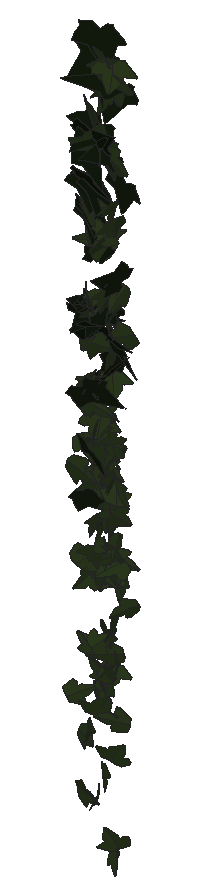
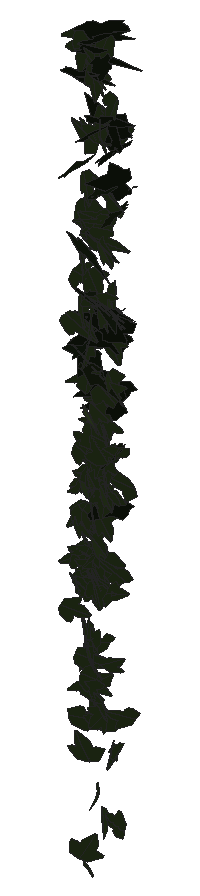
# SketchUp Ruby script. Lengths in inches.
U = 1.inch
M = Sketchup.active_model
def pt(a) = Geom::Point3d.new(a.map { |v| v * U })
def face(e, loops, mat)
  f = e.add_face(loops[0].map { |a| pt(a) })
  loops[1..].each { |l| e.add_face(l.map { |a| pt(a) }).erase! }
  f.material = f.back_material = mat if mat
  f
end
# faces: each face lists its corners as indices into pts; further lists are holes
def faces(e, pts, list, mat = nil) = list.each { |f| face(e, (f[0].is_a?(Array) ? f : [f]).map { |l| l.map { |i| pts[i] } }, mat) }
# xy, xz, yz: faces in a plane at the given z, y or x. An outline is a flat list of corners, or four numbers for a rectangle; further outlines are holes
def ring(l) = l.size == 4 ? [[l[0], l[1]], [l[2], l[1]], [l[2], l[3]], [l[0], l[3]]] : l.each_slice(2).to_a
def flat(e, list, mat, &to3) = list.each { |f| face(e, (f[0].is_a?(Array) ? f : [f]).map { |l| ring(l).map { |u, v| to3.(u, v) } }, mat) }
def xy(e, z, list, mat = nil) = flat(e, list, mat) { |x, y| [x, y, z] }
def xz(e, y, list, mat = nil) = flat(e, list, mat) { |x, z| [x, y, z] }
def yz(e, x, list, mat = nil) = flat(e, list, mat) { |y, z| [x, y, z] }
def lines(e, pts, list) = list.each { |a, b| e.add_line(pt(pts[a]), pt(pts[b])) }
# prism: a flat outline (further loops are holes) pulled along v
def prism(e, loops, v, mat = nil)
  f = face(e, loops, mat); d = Geom::Vector3d.new(v.map { |x| x * U })
  f.pushpull(f.normal.samedirection?(d) ? d.length : -d.length)
end
def box(e, o, s, mat = nil) = prism(e, [[o, [o[0] + s[0], o[1], o[2]], [o[0] + s[0], o[1] + s[1], o[2]], [o[0], o[1] + s[1], o[2]]]], [0, 0, s[2]], mat)
def at(x, y, z, deg = 0) = Geom::Transformation.translation(pt([x, y, z])) * Geom::Transformation.rotation(ORIGIN, Z_AXIS, deg.degrees)
def axes(o, x, y, z) = Geom::Transformation.new([*x, 0, *y, 0, *z, 0, *pt(o).to_a, 1])
def part(name) = M.definitions.add(name)
# library, detail: a bought-in or finely detailed component or shape, given as its bounding box
def library(name, o, s) = part(name).tap { |d| box(d.entities, o, s) }
def detail(e, o, s) = box(e.add_group.entities, o, s)
def put(e, d, t, mat = nil) = e.add_instance(d, t).tap { |i| i.material = mat if mat }
def group(e, t, mat = nil) = e.add_group.tap { |g| g.transformation = t; g.material = mat if mat }.entities
root = M.entities
M.materials.add("1026 AP 7946 SUNNY SIDE UP").color = [254, 231, 186]
M.materials.add("efeu1").color = [18, 25, 13]
M.materials.add("efeu2").color = [43, 57, 29]
c1 = part("ivyleaf_10")
p = [[0,0.5,-0.03],[-0.0625,2.02,-0.43],[-0.19,2.01,-0.46],[-0.54,1.05,-0.29],[-0.52,0.625,-0.18],[-0.83,0.76,-0.28],
  [-1.16,0.64,-0.33],[-1.15,0.33,-0.24],[-0.77,-0.39,0.02],[-0.3,-0.51,0.16],[0.04,-0.48,0.23],[-0.02,2.01,-0.4375],
  [-0.06,2.01,-0.43],[0.04,-0.49,0.23],[0.67,-0.49,0.14],[1.38,0.36,-0.2],[1.375,0.51,-0.24],[0.81,0.65,-0.19],
  [0.62,0.59,-0.15],[0.6,1.09,-0.28],[0.5,1.23,-0.31]]
faces(c1.entities,p,[[0,1,2,3,4,5,6,7,8,9,10],[11,12,0,13,14,15,16,17,18,19,20]],"efeu2")
c2 = part("ivyleaf_9")
p = [[1.54,2.16,1.25],[1.36,2.04,1.19],[-0.21,0.99,0.68],[-0.71,1.11,0.82],[-0.85,0.86,0.67],[-0.8,0.17,0.21],
  [-0.9,-0.01,0.1],[-0.67,-0.16,-0.02],[-0.08,-0.08,-0.05],[-0.03,-0.6,-0.4],[0.65,-0.88,-0.66],[0.83,-0.6,-0.49],
  [1.29,-0.42,-0.43],[1.8125,-0.07,-0.26],[1.21,0.44,0.15]]
faces(c2.entities,p,[[0,1,2,3,4,5,6,7,8,9,10,11,12,13,14]],"efeu1")
put(root,c1,axes([100.02,212.2,253.01],[0.11232,0.03435,-0.19191],[0.22416,0.12167,0.08006],[0.1966,-0.15835,0.01836]),"1026 AP 7946 SUNNY SIDE UP")
put(root,c1,axes([99.95,212.35,258.05],[-0.08901,-0.00971,-0.23971],[0.30282,-0.1365,-0.04321],[-0.20576,-0.19669,0.04011]),"1026 AP 7946 SUNNY SIDE UP")
put(root,c1,axes([100.17,212.54,261.8],[0.2145,-0.16612,0.0954],[0.07546,-0.08141,-0.22149],[0.29012,0.14399,-0.01293]),"1026 AP 7946 SUNNY SIDE UP")
put(root,c1,axes([100.38,212.41,261.08],[-0.3224,0.01429,0.10502],[-0.16795,-0.03042,-0.20113],[0.00238,-0.2115,0.03299]),"1026 AP 7946 SUNNY SIDE UP")
put(root,c1,axes([100.23,212.44,266.1875],[-0.2528,0.19125,-0.00279],[-0.00815,-0.01019,-0.25942],[-0.32467,-0.14866,0.00868]),"1026 AP 7946 SUNNY SIDE UP")
put(root,c2,axes([100.15,212.61,264.37],[-0.13446,-0.21379,0.0462],[0.07642,-0.06376,-0.23544],[0.36325,-0.06572,0.06663]),"1026 AP 7946 SUNNY SIDE UP")
put(root,c2,axes([99.98,212.4375,264.55],[0.30128,-0.08741,0.09348],[0.1197,-0.05623,-0.21174],[0.17389,0.19016,-0.0162]),"1026 AP 7946 SUNNY SIDE UP")
put(root,c2,axes([100.11,212.53,263.83],[0.04954,-0.18719,0.09598],[0.02599,-0.09082,-0.20409],[0.35319,0.03294,0.00155]),"1026 AP 7946 SUNNY SIDE UP")
put(root,c1,axes([100.3,212.43,255.68],[0.06854,0.08363,-0.19798],[-0.11915,-0.17724,-0.09796],[-0.30799,0.08718,-0.00616]),"1026 AP 7946 SUNNY SIDE UP")
put(root,c1,axes([100.41,212.21,262.04],[-0.17928,0.13464,0.16567],[-0.19153,0.10486,-0.18073],[-0.2881,-0.1535,0.01706]),"1026 AP 7946 SUNNY SIDE UP")
put(root,c1,axes([100.06,212.43,250.74],[-0.02848,-0.01566,0.21534],[0.3188,-0.05492,0.01353],[0.08422,0.20259,0.0216]),"1026 AP 7946 SUNNY SIDE UP")
put(root,c2,axes([99.99,212.49,261.4],[0.12929,-0.01929,0.21203],[0.32753,-0.0458,-0.08474],[0.08434,0.20743,0.00407]),"1026 AP 7946 SUNNY SIDE UP")
put(root,c2,axes([100.39,212.47,261.71],[-0.34952,-0.06685,-0.02328],[0.0448,-0.01402,-0.23082],[0.11011,-0.20648,0.02002]),"1026 AP 7946 SUNNY SIDE UP")
put(root,c2,axes([100.19,212.71,261.6],[-0.01809,-0.22466,0.10109],[-0.00817,-0.09927,-0.23232],[0.3862,-0.01262,-0.00018]),"1026 AP 7946 SUNNY SIDE UP")
put(root,c1,axes([100.4,212.5,260.01],[-0.18514,-0.14576,0.11913],[-0.0648,-0.114,-0.19057],[0.28613,-0.12013,0.03393]),"1026 AP 7946 SUNNY SIDE UP")
put(root,c1,axes([100.2,212.36,258.72],[0.17678,0.17856,0.05668],[0.06087,0.03935,-0.21682],[-0.28693,0.11835,-0.01108]),"1026 AP 7946 SUNNY SIDE UP")
put(root,c1,axes([100.32,212.59,257.91],[0.05907,-0.19507,0.03932],[0.01068,-0.03868,-0.20488],[0.3127,0.03817,-0.00043]),"1026 AP 7946 SUNNY SIDE UP")
put(root,c1,axes([100.32,212.63,263.15],[0.05356,-0.20375,0.07156],[0.02363,-0.06816,-0.22166],[0.36468,0.03434,0.00385]),"1026 AP 7946 SUNNY SIDE UP")
put(root,c1,axes([100.3,212.17,252.24],[-0.0456,0.16963,0.1193],[-0.03498,0.1127,-0.17661],[-0.3202,-0.03647,0.0023]),"1026 AP 7946 SUNNY SIDE UP")
put(root,c1,axes([100.35,212.34,260.2],[0.01854,-0.22025,0.02777],[0.00192,-0.02818,-0.22739],[0.34915,0.01185,-0.00023]),"1026 AP 7946 SUNNY SIDE UP")
put(root,c2,axes([100.1875,212.42,265.18],[0.06286,-0.2409,-0.05369],[-0.00403,0.051,-0.2512],[0.38709,0.03965,0.00611]),"1026 AP 7946 SUNNY SIDE UP")
put(root,c1,axes([100.46,212.38,254.07],[0.19071,0.08353,0.11644],[-0.17863,-0.0355,0.14653],[0.147,-0.15151,0.02699]),"1026 AP 7946 SUNNY SIDE UP")
put(root,c2,axes([100.43,212.52,265.8],[-0.34827,-0.11379,0.01185],[-0.00129,-0.02489,-0.25569],[0.17993,-0.22042,0.0211]),"1026 AP 7946 SUNNY SIDE UP")
put(root,c1,axes([100.57,212.56,263.26],[0.14508,-0.01975,-0.22507],[-0.34388,-0.0251,-0.09301],[-0.02446,0.23572,-0.02735]),"1026 AP 7946 SUNNY SIDE UP")
put(root,c1,axes([100.37,212.49,261.67],[-0.02837,-0.23276,0.01754],[0.00083,-0.01844,-0.24061],[0.36713,-0.01794,0.0019]),"1026 AP 7946 SUNNY SIDE UP")
put(root,c1,axes([100.35,212.28,252.28],[0.04208,-0.12091,-0.17236],[0.01402,0.16854,-0.12354],[0.3234,0.00843,0.02778]),"1026 AP 7946 SUNNY SIDE UP")
put(root,c1,axes([100.37,212.51,258.28],[0.10936,-0.19314,-0.06257],[0.01146,0.06078,-0.21551],[0.34115,0.05987,0.0273]),"1026 AP 7946 SUNNY SIDE UP")
put(root,c2,axes([100.54,212.39,261.85],[-0.00915,0.2195,0.09172],[-0.10688,0.07844,-0.22589],[-0.38364,-0.02709,0.06074]),"1026 AP 7946 SUNNY SIDE UP")
put(root,c1,axes([100.16,212.32,256.01],[0.26402,0.00409,-0.15919],[0.24034,0.02989,0.17206],[0.03653,-0.22624,0.01851]),"1026 AP 7946 SUNNY SIDE UP")
put(root,c2,axes([100.22,212.42,258.63],[0.14458,-0.19886,0.0146],[0.00087,-0.01743,-0.23175],[0.3387,0.08493,-0.00564]),"1026 AP 7946 SUNNY SIDE UP")
put(root,c2,axes([100.26,212.32,257.57],[0.01233,-0.06509,-0.21997],[0.02946,0.20424,-0.06605],[0.36331,-0.01435,0.01282]),"1026 AP 7946 SUNNY SIDE UP")
put(root,c1,axes([100.4,212.4375,257.73],[-0.20995,-0.16702,-0.04125],[0.05473,0.02213,-0.21974],[0.26412,-0.13735,0.01275]),"1026 AP 7946 SUNNY SIDE UP")
put(root,c2,axes([100.31,212.51,263.76],[-0.05792,-0.21022,0.08986],[0.0023,-0.08783,-0.22872],[0.38599,-0.03102,0.01485]),"1026 AP 7946 SUNNY SIDE UP")
put(root,c2,axes([100.21,212.45,265.3125],[-0.01613,0.0612,0.25776],[0.1332,-0.23531,0.06158],[0.38194,0.08465,-0.01059]),"1026 AP 7946 SUNNY SIDE UP")
put(root,c2,axes([100.15,212.37,259.76],[0.31643,-0.08239,0.06881],[0.08995,-0.04129,-0.21812],[0.1542,0.19316,-0.01396]),"1026 AP 7946 SUNNY SIDE UP")
put(root,c1,axes([100.36,212.55,258.61],[-0.11161,-0.19546,0.06933],[0.03319,0.06511,0.2146],[-0.32393,0.07402,-0.0019]),"1026 AP 7946 SUNNY SIDE UP")
put(root,c1,axes([100.23,212.54,257.91],[0.23126,-0.02314,0.16106],[0.23206,-0.05679,-0.15189],[0.08947,0.20709,-0.02234]),"1026 AP 7946 SUNNY SIDE UP")
put(root,c1,axes([100.41,212.36,265.37],[-0.32377,-0.18979,0.03198],[0.02012,0.03344,0.28822],[-0.30201,0.2057,-0.01509]),"1026 AP 7946 SUNNY SIDE UP")
put(root,c1,axes([100.48,212.625,259.68],[-0.00518,-0.1834,0.14435],[0.01457,-0.14117,-0.18955],[0.36363,0.00304,0.00965]),"1026 AP 7946 SUNNY SIDE UP")
put(root,c1,axes([100.46,212.5,258.53],[-0.34133,0.04572,-0.02261],[0.02625,-0.02924,-0.21954],[-0.08182,-0.20011,0.02392]),"1026 AP 7946 SUNNY SIDE UP")
put(root,c1,axes([100.5,212.38,256.33],[-0.24778,-0.14408,-0.00158],[0.01713,-0.01085,-0.21946],[0.22591,-0.15721,0.0149]),"1026 AP 7946 SUNNY SIDE UP")
put(root,c1,axes([100.2,212.39,263.97],[0.11901,-0.12099,-0.2365],[0.28652,-0.1445,0.13992],[-0.28918,-0.19297,0.04131]),"1026 AP 7946 SUNNY SIDE UP")
put(root,c2,axes([100.36,212.56,264.28],[-0.07832,-0.1897,0.14558],[0.05643,-0.14985,-0.1936],[0.36866,-0.01736,0.06056]),"1026 AP 7946 SUNNY SIDE UP")
put(root,c1,axes([100.52,212.35,250.85],[0.04542,-0.17403,-0.13453],[-0.02541,0.12866,-0.18093],[0.34024,0.03284,0.00445]),"1026 AP 7946 SUNNY SIDE UP")
put(root,c1,axes([100.43,212.41,259.11],[0.14879,-0.19319,0.04233],[0.07543,-0.02558,-0.22529],[0.32704,0.09379,0.0327]),"1026 AP 7946 SUNNY SIDE UP")
put(root,c1,axes([100.62,212.39,253.18],[0.02992,-0.0335,-0.20528],[-0.16171,0.17045,-0.03868],[0.27314,0.10459,-0.00042]),"1026 AP 7946 SUNNY SIDE UP")
put(root,c1,axes([100.45,212.39,267.49],[-0.32438,0.16486,-0.0372],[0.03239,-0.03429,-0.27028],[-0.28494,-0.19157,0.01162]),"1026 AP 7946 SUNNY SIDE UP")
put(root,c1,axes([100.51,212.59,255.71],[-0.18964,-0.1365,0.0365],[0.01615,-0.05293,-0.18464],[0.23904,-0.10472,0.04143]),"1026 AP 7946 SUNNY SIDE UP")
put(root,c2,axes([100.29,212.57,267.1],[0.31066,-0.15795,-0.01776],[-0.03737,-0.00332,-0.25822],[0.26666,0.18355,-0.0155]),"1026 AP 7946 SUNNY SIDE UP")
put(root,c1,axes([100.51,212.54,261.95],[0.25058,0.11101,-0.10091],[-0.10851,-0.07348,-0.19782],[-0.2239,0.15985,-0.01707]),"1026 AP 7946 SUNNY SIDE UP")
put(root,c2,axes([100.6,212.49,267.45],[-0.294,-0.16201,0.15279],[-0.11493,-0.13902,-0.25064],[0.32673,-0.19469,0.04932]),"1026 AP 7946 SUNNY SIDE UP")
put(root,c2,axes([100.4,212.59,267.87],[-0.14933,-0.2332,-0.10196],[0.0647,0.08866,-0.25885],[0.39224,-0.10341,0.00388]),"1026 AP 7946 SUNNY SIDE UP")
put(root,c1,axes([100.49,212.61,256.79],[0.06669,-0.18204,0.11534],[0.04807,-0.10886,-0.19314],[0.33345,0.0521,0.00478]),"1026 AP 7946 SUNNY SIDE UP")
put(root,c2,axes([100.25,212.28,261.23],[0.37433,0.05443,0.11268],[0.17439,0.00258,-0.25069],[-0.07953,0.26184,-0.01935]),"1026 AP 7946 SUNNY SIDE UP")
put(root,c1,axes([100.54,212.59,255.82],[-0.09718,-0.1693,0.03564],[0.03557,-0.04391,-0.1886],[0.29149,-0.05109,0.0349]),"1026 AP 7946 SUNNY SIDE UP")
put(root,c2,axes([100.54,212.34,262.97],[-0.24996,0.18008,-0.00187],[0.01049,0.01034,0.24888],[0.30559,0.14694,-0.01007]),"1026 AP 7946 SUNNY SIDE UP")
put(root,c2,axes([100.29,212.38,265.49],[-0.06415,-0.04601,0.25204],[0.27447,-0.18171,-0.01275],[0.30215,0.15529,0.06509]),"1026 AP 7946 SUNNY SIDE UP")
put(root,c1,axes([100.57,212.34,257.09],[-0.02611,-0.19826,0.06145],[-0.00206,-0.06087,-0.20529],[0.32606,-0.01626,0.00363]),"1026 AP 7946 SUNNY SIDE UP")
put(root,c2,axes([100.72,212.53,260.38],[-0.21941,0.16933,-0.05677],[-0.01095,-0.07265,-0.2233],[-0.30216,-0.12033,0.04931]),"1026 AP 7946 SUNNY SIDE UP")
put(root,c1,axes([100.4,212.57,265.44],[0.15237,-0.12165,0.19296],[0.20904,-0.13435,-0.16318],[0.30694,0.15188,0.01534]),"1026 AP 7946 SUNNY SIDE UP")
put(root,c1,axes([100.58,212.49,258.12],[-0.1544,-0.16706,0.06674],[0.01876,-0.08083,-0.19375],[0.28167,-0.08619,0.04949]),"1026 AP 7946 SUNNY SIDE UP")
put(root,c2,axes([100.59,212.45,261.76],[-0.3382,-0.03188,-0.09592],[0.15731,-0.02272,-0.21325],[0.0332,-0.21709,0.03327]),"1026 AP 7946 SUNNY SIDE UP")
put(root,c1,axes([100.47,212.51,253.02],[-0.23361,0.1164,-0.09158],[0.09623,-0.06674,-0.19433],[-0.20992,-0.16012,0.01283]),"1026 AP 7946 SUNNY SIDE UP")
put(root,c2,axes([100.38,212.125,260.05],[0.02233,-0.02652,-0.25259],[0.08821,0.23054,-0.02146],[0.39267,-0.05028,0.01919]),"1026 AP 7946 SUNNY SIDE UP")
put(root,c1,axes([100.32,212.28,259.67],[-0.12724,-0.02671,-0.21996],[0.33435,-0.04384,-0.07768],[-0.05028,-0.22394,0.04007]),"1026 AP 7946 SUNNY SIDE UP")
put(root,c1,axes([100.52,212.42,259.24],[0.36147,0.05157,-0.00551],[-0.00047,-0.02344,-0.23362],[-0.0881,0.21172,-0.02136]),"1026 AP 7946 SUNNY SIDE UP")
put(root,c1,axes([100.76,212.375,253.57],[-0.22959,0.01286,-0.14556],[-0.21771,0.03177,0.1505],[0.04917,0.20073,-0.01329]),"1026 AP 7946 SUNNY SIDE UP")
put(root,c1,axes([100.61,212.54,266.75],[-0.04848,-0.24168,-0.06331],[0.01106,0.0556,-0.25976],[0.42097,-0.02929,-0.00047]),"1026 AP 7946 SUNNY SIDE UP")
put(root,c1,axes([100.53,212.55,251.35],[-0.05325,0.16043,-0.12883],[0.0335,-0.12421,-0.16959],[-0.31897,-0.03983,0.0037]),"1026 AP 7946 SUNNY SIDE UP")
put(root,c2,axes([100.93,212.37,267.02],[-0.33794,0.03228,0.1539],[-0.24831,-0.02091,-0.21276],[-0.02339,-0.24442,0.03503]),"1026 AP 7946 SUNNY SIDE UP")
put(root,c2,axes([100.87,212.52,261.88],[-0.33066,0.10854,0.05356],[-0.08717,0.00738,-0.23783],[-0.1821,-0.20063,0.0166]),"1026 AP 7946 SUNNY SIDE UP")
put(root,c1,axes([100.68,212.41,258.65],[-0.32666,-0.0896,0.00428],[0.00684,-0.02083,-0.22647],[0.1522,-0.19137,0.01936]),"1026 AP 7946 SUNNY SIDE UP")
put(root,c1,axes([100.67,212.5625,257.94],[0.12153,-0.19484,-0.03182],[-0.02381,0.02602,-0.21574],[0.30901,0.07864,-0.00411]),"1026 AP 7946 SUNNY SIDE UP")
put(root,c1,axes([100.78,212.43,257.29],[-0.10748,0.0944,0.17248],[-0.21476,0.10169,-0.11651],[-0.23068,-0.13866,0.02811]),"1026 AP 7946 SUNNY SIDE UP")
put(root,c1,axes([100.59,212.29,252.73],[-0.32834,-0.06197,0.07208],[0.09669,0.03903,0.22377],[-0.11123,0.21685,-0.01826]),"1026 AP 7946 SUNNY SIDE UP")
put(root,c1,axes([100.59,212.28,256.35],[0.01027,-0.07594,-0.23259],[0.13323,0.21137,-0.06962],[0.34936,-0.07837,0.03338]),"1026 AP 7946 SUNNY SIDE UP")
put(root,c1,axes([100.77,212.4,261.49],[-0.11113,0.1091,0.20775],[-0.18885,0.15746,-0.13375],[-0.32491,-0.12884,0.00669]),"1026 AP 7946 SUNNY SIDE UP")
put(root,c1,axes([100.67,212.51,258.11],[0.03255,-0.19187,0.06888],[0.02857,-0.06628,-0.19891],[0.31877,0.02553,0.0108]),"1026 AP 7946 SUNNY SIDE UP")
put(root,c1,axes([100.57,212.65,254.21],[0.21992,-0.12288,0.13831],[0.13067,-0.1085,-0.19113],[0.25551,0.16125,-0.0213]),"1026 AP 7946 SUNNY SIDE UP")
put(root,c1,axes([100.5,212.49,258.3],[-0.2255,0.00458,-0.17077],[0.25115,-0.05524,-0.14423],[-0.07026,-0.21214,0.03254]),"1026 AP 7946 SUNNY SIDE UP")
put(root,c1,axes([100.7,212.59,257.3],[-0.00209,-0.17361,0.14066],[0.02455,-0.13726,-0.17916],[0.34739,0.00866,0.01351]),"1026 AP 7946 SUNNY SIDE UP")
put(root,c1,axes([100.64,212.25,263.13],[0.04097,-0.10277,0.23674],[-0.01647,0.22298,0.11451],[-0.41568,-0.01896,0.0188]),"1026 AP 7946 SUNNY SIDE UP")
put(root,c1,axes([100.74,212.48,255.9],[0.11632,-0.16526,-0.06925],[-0.04881,0.05574,-0.19067],[0.29594,0.07415,-0.00423]),"1026 AP 7946 SUNNY SIDE UP")
put(root,c2,axes([100.79,212.5,265.3],[-0.20618,-0.08332,0.1974],[-0.15059,-0.17768,-0.14779],[0.29277,-0.15007,0.063]),"1026 AP 7946 SUNNY SIDE UP")
put(root,c1,axes([100.74,212.56,255.83],[0.30846,0.00362,-0.06745],[-0.1018,-0.02241,-0.20119],[-0.01653,0.2056,-0.01953]),"1026 AP 7946 SUNNY SIDE UP")
put(root,c1,axes([100.65,212.45,255.96],[0.14059,-0.14047,0.1013],[0.08133,-0.08373,-0.17575],[0.2776,0.09567,0.00018]),"1026 AP 7946 SUNNY SIDE UP")
put(root,c1,axes([100.61,212.19,261.09],[-0.06901,-0.10611,-0.20795],[0.1695,0.16589,-0.11793],[0.33301,-0.10643,0.01693]),"1026 AP 7946 SUNNY SIDE UP")
put(root,c1,axes([100.55,212.63,259.26],[-0.02077,-0.09756,-0.18025],[0.15477,-0.15059,0.08488],[-0.28972,-0.07345,0.05826]),"1026 AP 7946 SUNNY SIDE UP")
put(root,c1,axes([100.5,212.3125,263.41],[0.08255,0.01522,-0.24501],[0.29318,0.15182,0.05218],[0.25672,-0.17828,0.0192]),"1026 AP 7946 SUNNY SIDE UP")
put(root,c1,axes([100.72,212.61,253.84],[-0.0405,-0.119,0.19934],[0.04048,-0.19568,-0.12117],[0.3558,0.00872,0.03647]),"1026 AP 7946 SUNNY SIDE UP")
put(root,c1,axes([100.73,212.46,258.77],[-0.22442,-0.15011,-0.0218],[-0.03076,-0.00855,0.21386],[-0.25488,0.13321,-0.00661]),"1026 AP 7946 SUNNY SIDE UP")
put(root,c1,axes([100.71,212.4375,266.69],[0.2798,-0.17346,0.0382],[0.02285,-0.03941,-0.25606],[0.30055,0.16448,-0.01609]),"1026 AP 7946 SUNNY SIDE UP")
put(root,c1,axes([100.93,212.44,254.1],[-0.06143,-0.02336,0.21441],[-0.23676,-0.14421,-0.04661],[0.22918,-0.15524,0.00932]),"1026 AP 7946 SUNNY SIDE UP")
put(root,c1,axes([100.64,212.14,254.36],[0.10131,0.04791,-0.19335],[0.15676,0.16171,0.07862],[0.26162,-0.11544,0.02776]),"1026 AP 7946 SUNNY SIDE UP")
put(root,c1,axes([100.72,212.59,253.64],[0.23143,0.1405,-0.04984],[-0.04058,-0.04403,-0.20941],[-0.23053,0.1488,-0.01318]),"1026 AP 7946 SUNNY SIDE UP")
put(root,c2,axes([100.82,212.61,260.66],[-0.31486,0.04965,-0.10938],[0.15412,-0.05479,-0.20444],[-0.11753,-0.20487,0.02493]),"1026 AP 7946 SUNNY SIDE UP")
put(root,c1,axes([100.72,212.41,253.36],[0.26453,-0.11554,0.04044],[0.03856,-0.03461,-0.20993],[0.1883,0.16941,-0.01382]),"1026 AP 7946 SUNNY SIDE UP")
put(root,c1,axes([100.85,212.58,257.31],[-0.1284,-0.18466,0.09308],[-0.04058,-0.08838,-0.20821],[0.32143,-0.08492,0.0109]),"1026 AP 7946 SUNNY SIDE UP")
put(root,c1,axes([100.8125,212.36,262.23],[-0.05642,-0.22314,0.0555],[-0.00084,-0.05573,-0.23301],[0.36142,-0.03497,0.00812]),"1026 AP 7946 SUNNY SIDE UP")
put(root,c1,axes([100.77,212.43,256.43],[-0.30054,0.1265,-0.0234],[0.01391,-0.02895,-0.23547],[-0.20182,-0.19038,0.01863]),"1026 AP 7946 SUNNY SIDE UP")
put(root,c1,axes([100.8,212.51,257.96],[0.0003,-0.17489,0.10844],[0.01547,-0.10612,-0.18058],[0.32139,0.00527,0.00859]),"1026 AP 7946 SUNNY SIDE UP")
put(root,c1,axes([100.78,212.44,260.82],[0.05403,-0.16406,-0.15755],[0.0384,0.15561,-0.16644],[0.34956,0.00827,0.04264]),"1026 AP 7946 SUNNY SIDE UP")
put(root,c1,axes([100.69,212.31,263.47],[0.14357,0.1093,-0.19704],[0.14836,0.16843,0.14607],[0.31395,-0.12957,0.02108]),"1026 AP 7946 SUNNY SIDE UP")
put(root,c1,axes([100.85,212.5,257.2],[-0.14343,-0.17574,0.06999],[-0.01893,-0.07099,-0.20327],[0.29623,-0.08963,0.02089]),"1026 AP 7946 SUNNY SIDE UP")
put(root,c1,axes([100.87,212.36,267.39],[-0.23791,-0.20145,0.03871],[-0.01748,-0.04,-0.26285],[0.34782,-0.1398,0.01326]),"1026 AP 7946 SUNNY SIDE UP")
put(root,c1,axes([100.73,212.57,260.22],[0.19746,0.18135,-0.0201],[0.00094,-0.02541,-0.23052],[-0.30994,0.11546,-0.0135]),"1026 AP 7946 SUNNY SIDE UP")
put(root,c1,axes([100.74,212.67,258],[0.08328,-0.12449,0.18389],[0.12042,-0.16208,-0.14025],[0.32128,0.09301,0.0049]),"1026 AP 7946 SUNNY SIDE UP")
put(root,c2,axes([100.81,212.65,266.72],[-0.31722,-0.13544,-0.07609],[0.13146,0.00472,-0.24673],[0.20317,-0.21452,0.04085]),"1026 AP 7946 SUNNY SIDE UP")
put(root,c1,axes([100.59,212.37,255.97],[0.14293,-0.00948,0.19259],[0.28955,-0.03309,-0.09414],[0.05328,0.20527,-0.00504]),"1026 AP 7946 SUNNY SIDE UP")
put(root,c1,axes([100.875,212.49,254.8125],[0.11843,-0.16892,-0.10788],[-0.03049,0.10419,-0.18863],[0.31022,0.07473,0.02265]),"1026 AP 7946 SUNNY SIDE UP")
put(root,c1,axes([100.89,212.59,258.63],[-0.04709,-0.1575,0.14358],[-0.01506,-0.14051,-0.16546],[0.33128,-0.02877,0.01289]),"1026 AP 7946 SUNNY SIDE UP")
put(root,c1,axes([100.67,212.43,254.47],[-0.12685,0.04055,0.18944],[0.25819,-0.08228,0.09254],[0.14423,0.18295,0.00096]),"1026 AP 7946 SUNNY SIDE UP")
put(root,c1,axes([100.875,212.33,254.72],[0.01449,-0.12557,-0.16425],[0.00209,0.15892,-0.12852],[0.31824,0.00467,0.00832]),"1026 AP 7946 SUNNY SIDE UP")
put(root,c1,axes([100.875,212.45,263.76],[-0.08528,-0.24481,-0.04122],[0.02956,0.03535,-0.25788],[0.38858,-0.05642,0.01057]),"1026 AP 7946 SUNNY SIDE UP")
put(root,c1,axes([100.88,212.53,261.76],[0.02243,-0.2192,-0.06425],[0.01651,0.05775,-0.23389],[0.38419,0.01031,0.0138]),"1026 AP 7946 SUNNY SIDE UP")
put(root,c1,axes([100.72,212.4,256.09],[0.13883,0.11287,0.13655],[0.12477,0.10243,-0.14779],[-0.25874,0.10996,0.002]),"1026 AP 7946 SUNNY SIDE UP")
put(root,c1,axes([100.88,212.6,257.14],[0.02139,-0.21651,0.11193],[0.03742,-0.10833,-0.22358],[0.37993,0.02286,0.01572]),"1026 AP 7946 SUNNY SIDE UP")
put(root,c1,axes([101.0625,212.35,256.21],[-0.29732,0.08392,0.0888],[-0.19595,-0.14916,-0.10278],[0.03476,-0.123,0.1802]),"1026 AP 7946 SUNNY SIDE UP")
put(root,c1,axes([100.83,212.38,255.88],[-0.17056,-0.13886,-0.10331],[0.12033,0.06587,-0.18027],[0.24015,-0.13163,0.01695]),"1026 AP 7946 SUNNY SIDE UP")
put(root,c1,axes([100.99,212.39,249.86],[-0.21845,-0.11564,-0.10571],[-0.14379,-0.04867,0.18496],[-0.19515,0.1653,-0.01796]),"1026 AP 7946 SUNNY SIDE UP")
put(root,c1,axes([101.13,212.56,261.29],[-0.19767,0.01166,0.19454],[-0.28735,-0.0659,-0.12157],[0.07664,-0.21702,0.04598]),"1026 AP 7946 SUNNY SIDE UP")
put(root,c1,axes([100.97,212.41,256.21],[-0.18678,-0.16507,0.04926],[-0.02271,-0.04948,-0.20909],[0.26968,-0.11849,0.01652]),"1026 AP 7946 SUNNY SIDE UP")
put(root,c1,axes([100.92,212.32,267.05],[-0.41091,0.04975,-0.02463],[0.03047,-0.02954,-0.26359],[-0.0884,-0.24141,0.02361]),"1026 AP 7946 SUNNY SIDE UP")
put(root,c2,axes([100.96,212.1875,260.54],[0.07082,0.19608,0.14881],[0.06417,0.13759,-0.20632],[-0.37648,0.06034,-0.00717]),"1026 AP 7946 SUNNY SIDE UP")
put(root,c1,axes([100.95,212.29,258.1],[0.09254,-0.19434,-0.04089],[-0.00759,0.03884,-0.20886],[0.31146,0.05869,0.00706]),"1026 AP 7946 SUNNY SIDE UP")
put(root,c1,axes([100.95,212.35,264.27],[0.01599,-0.24069,-0.02904],[0.01726,0.02728,-0.24771],[0.38041,0.00888,0.01246]),"1026 AP 7946 SUNNY SIDE UP")
put(root,c2,axes([100.76,212.62,260.92],[0.18097,-0.18285,0.04169],[0.02062,-0.04071,-0.22692],[0.31755,0.10685,-0.00902]),"1026 AP 7946 SUNNY SIDE UP")
put(root,c1,axes([101.17,212.35,252.6875],[0.01253,0.02647,0.2072],[-0.26634,-0.10962,0.02115],[0.17511,-0.16864,0.01735]),"1026 AP 7946 SUNNY SIDE UP")
put(root,c1,axes([100.8125,212.46,257.87],[-0.20789,0.06619,-0.154],[0.19396,-0.08652,-0.15198],[-0.16954,-0.18015,0.01496]),"1026 AP 7946 SUNNY SIDE UP")
put(root,c1,axes([100.99,212.35,257.66],[0.14262,0.18727,-0.06641],[0.01193,0.06872,0.21356],[0.31175,-0.08831,0.02221]),"1026 AP 7946 SUNNY SIDE UP")
put(root,c2,axes([101.24,212.16,262.71],[-0.21579,0.21999,0.07746],[-0.08026,0.05519,-0.26642],[-0.35599,-0.14579,0.01311]),"1026 AP 7946 SUNNY SIDE UP")
put(root,c1,axes([100.9375,212.31,267.38],[0.32653,0.14891,-0.0262],[-0.01488,-0.03176,-0.26261],[-0.2373,0.20689,-0.01958]),"1026 AP 7946 SUNNY SIDE UP")
put(root,c1,axes([100.92,212.59,255.7],[0.24874,-0.0846,0.08778],[0.10656,-0.05673,-0.18113],[0.17078,0.15861,-0.01483]),"1026 AP 7946 SUNNY SIDE UP")
put(root,c1,axes([100.97,212.38,257.25],[-0.10527,-0.14014,-0.1581],[0.1222,0.13175,-0.15893],[0.30208,-0.10214,0.0092]),"1026 AP 7946 SUNNY SIDE UP")
put(root,c1,axes([101.05,212.35,262.58],[0.16695,-0.20121,-0.06049],[-0.00428,0.06322,-0.23243],[0.32905,0.10291,0.02766]),"1026 AP 7946 SUNNY SIDE UP")
put(root,c1,axes([100.97,212.42,256.72],[0.21316,-0.12446,0.099],[0.08729,-0.08181,-0.18893],[0.23204,0.1451,-0.01987]),"1026 AP 7946 SUNNY SIDE UP")
put(root,c1,axes([100.79,212.41,265.21],[-0.01931,-0.00639,-0.28375],[0.28161,-0.20964,-0.00444],[-0.32912,-0.17901,0.01285]),"1026 AP 7946 SUNNY SIDE UP")
put(root,c1,axes([100.88,212.4,256.32],[-0.15712,-0.08511,-0.17914],[0.25931,0.06406,-0.12992],[0.15815,-0.1896,0.03506]),"1026 AP 7946 SUNNY SIDE UP")
put(root,c1,axes([101.05,212.47,262.28],[-0.0995,-0.13647,0.18951],[0.06002,-0.1952,-0.13623],[0.35611,-0.00523,0.07591]),"1026 AP 7946 SUNNY SIDE UP")
put(root,c1,axes([101.16,212.64,255.16],[-0.05285,-0.0831,0.18736],[-0.0886,-0.17351,-0.09317],[0.30237,-0.06537,0.00545]),"1026 AP 7946 SUNNY SIDE UP")
put(root,c1,axes([101.01,212.24,251.89],[-0.29688,-0.05156,0.07433],[0.10356,0.03314,0.20132],[-0.09393,0.19949,-0.01296]),"1026 AP 7946 SUNNY SIDE UP")
put(root,c2,axes([100.98,212.65,264.6],[-0.05428,-0.20989,0.1168],[0.01533,-0.11689,-0.21828],[0.37568,-0.02556,0.02578]),"1026 AP 7946 SUNNY SIDE UP")
put(root,c1,axes([101.13,212.17,254.04],[0.04813,-0.08763,-0.19606],[-0.02636,0.19019,-0.09213],[0.32768,0.02817,0.02139]),"1026 AP 7946 SUNNY SIDE UP")
put(root,c1,axes([100.95,212.35,249.67],[0.16399,-0.0774,0.1662],[0.18614,-0.11086,-0.13392],[0.21182,0.15734,-0.01099]),"1026 AP 7946 SUNNY SIDE UP")
